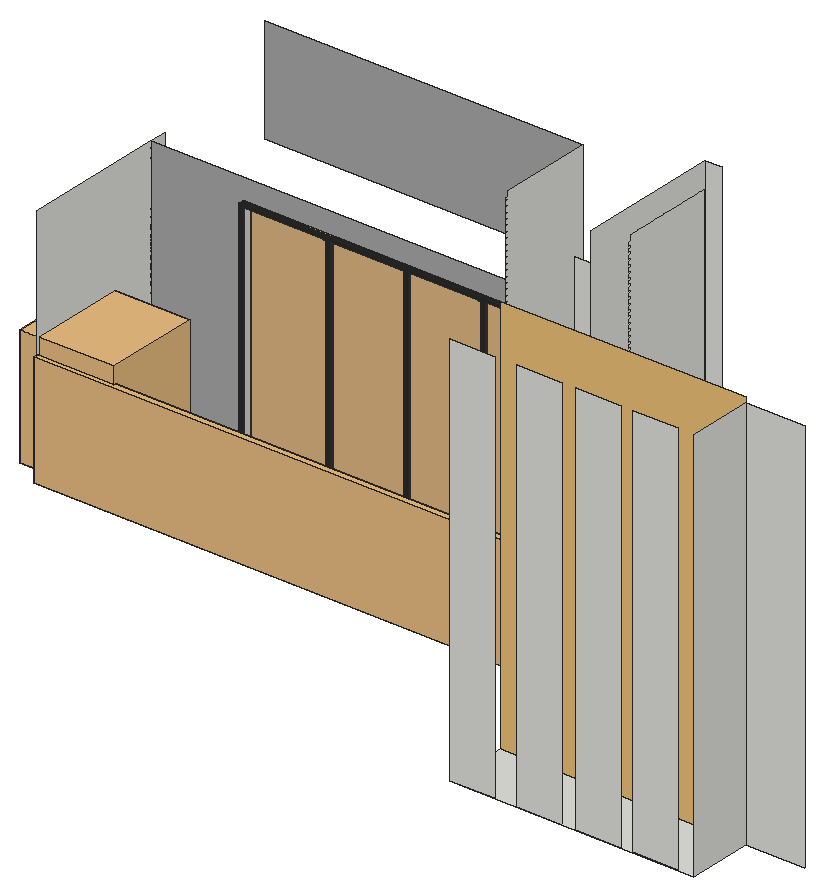
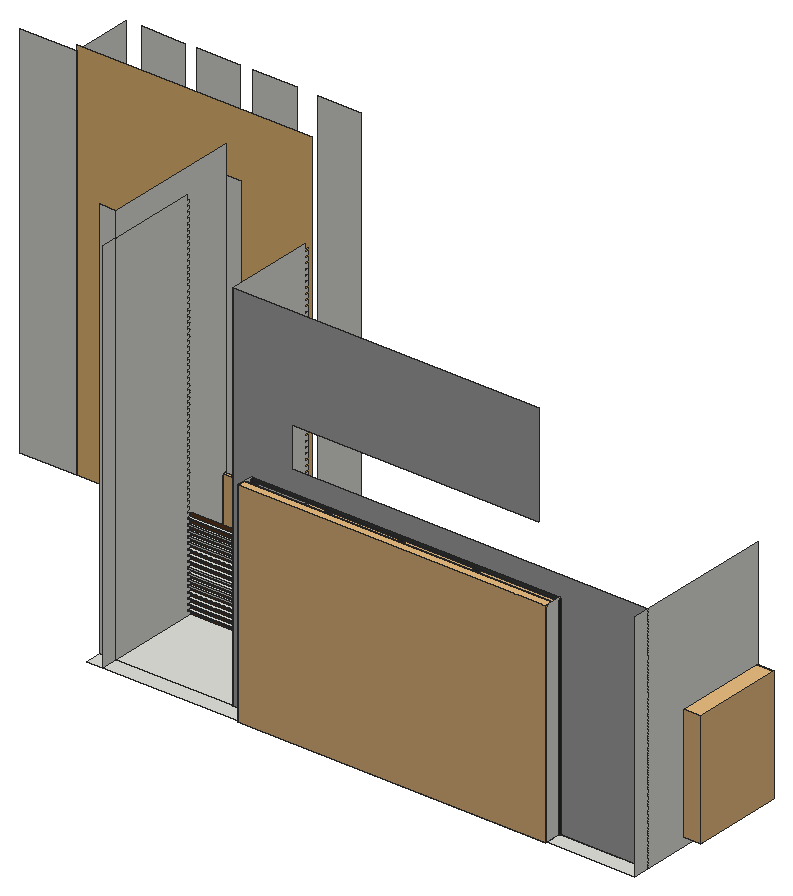
# SketchUp Ruby script. Lengths in inches.
U = 1.inch
M = Sketchup.active_model
def pt(a) = Geom::Point3d.new(a.map { |v| v * U })
def face(e, loops, mat)
  f = e.add_face(loops[0].map { |a| pt(a) })
  loops[1..].each { |l| e.add_face(l.map { |a| pt(a) }).erase! }
  f.material = f.back_material = mat if mat
  f
end
# faces: each face lists its corners as indices into pts; further lists are holes
def faces(e, pts, list, mat = nil) = list.each { |f| face(e, (f[0].is_a?(Array) ? f : [f]).map { |l| l.map { |i| pts[i] } }, mat) }
# xy, xz, yz: faces in a plane at the given z, y or x. An outline is a flat list of corners, or four numbers for a rectangle; further outlines are holes
def ring(l) = l.size == 4 ? [[l[0], l[1]], [l[2], l[1]], [l[2], l[3]], [l[0], l[3]]] : l.each_slice(2).to_a
def flat(e, list, mat, &to3) = list.each { |f| face(e, (f[0].is_a?(Array) ? f : [f]).map { |l| ring(l).map { |u, v| to3.(u, v) } }, mat) }
def xy(e, z, list, mat = nil) = flat(e, list, mat) { |x, y| [x, y, z] }
def xz(e, y, list, mat = nil) = flat(e, list, mat) { |x, z| [x, y, z] }
def yz(e, x, list, mat = nil) = flat(e, list, mat) { |y, z| [x, y, z] }
def lines(e, pts, list) = list.each { |a, b| e.add_line(pt(pts[a]), pt(pts[b])) }
# prism: a flat outline (further loops are holes) pulled along v
def prism(e, loops, v, mat = nil)
  f = face(e, loops, mat); d = Geom::Vector3d.new(v.map { |x| x * U })
  f.pushpull(f.normal.samedirection?(d) ? d.length : -d.length)
end
def box(e, o, s, mat = nil) = prism(e, [[o, [o[0] + s[0], o[1], o[2]], [o[0] + s[0], o[1] + s[1], o[2]], [o[0], o[1] + s[1], o[2]]]], [0, 0, s[2]], mat)
def at(x, y, z, deg = 0) = Geom::Transformation.translation(pt([x, y, z])) * Geom::Transformation.rotation(ORIGIN, Z_AXIS, deg.degrees)
def axes(o, x, y, z) = Geom::Transformation.new([*x, 0, *y, 0, *z, 0, *pt(o).to_a, 1])
def part(name) = M.definitions.add(name)
# library, detail: a bought-in or finely detailed component or shape, given as its bounding box
def library(name, o, s) = part(name).tap { |d| box(d.entities, o, s) }
def detail(e, o, s) = box(e.add_group.entities, o, s)
def put(e, d, t, mat = nil) = e.add_instance(d, t).tap { |i| i.material = mat if mat }
def group(e, t, mat = nil) = e.add_group.tap { |g| g.transformation = t; g.material = mat if mat }.entities
root = M.entities
M.materials.add("Glazing").color = [128, 128, 128]
M.materials["Glazing"].alpha = 0.05
M.materials.add("Powdercoating").color = [41, 44, 40]
M.materials.add("[Color M03]1").color = [170, 170, 170]
M.materials.add("[Wood OSB]1").color = [240, 195, 122]
M.materials.add("[Wood Veneer 01]").color = [96, 56, 29]
c1 = library("plant (1)",[-35.72,-28.42,0],[66.31,67.39,84.38])
c2 = part("Group\#15")
xy(c2.entities,0,[[0,-55.94,0.71,45.94]])
xy(c2.entities,0.2,[[0,-55.94,0.47,45.94],[0.47,45.94,0.71,46.42]])
xy(c2.entities,2.36,[[0.47,-55.94,0.71,46.42]])
xz(c2.entities,-55.94,[[0,0,0.71,0,0.71,2.36,0.47,2.36,0.47,0.2,0,0.2]])
xz(c2.entities,45.94,[[0,0,0.71,0.2]])
xz(c2.entities,46.42,[[0.47,0.2,0.71,2.36]])
yz(c2.entities,0,[[-55.94,0,45.94,0.2]])
yz(c2.entities,0.47,[[-55.94,0.2,46.42,2.36]])
yz(c2.entities,0.71,[[-55.94,0,45.94,0,45.94,0.2,46.42,0.2,46.42,2.36,-55.94,2.36]])
c3 = part("Group\#7")
xy(c3.entities,0,[[0,-59.09,0.71,45.94]])
xy(c3.entities,0.2,[[0,-59.09,0.47,45.94],[0.47,45.94,0.71,46.42]])
xy(c3.entities,2.36,[[0.47,-59.09,0.71,46.42]])
xz(c3.entities,-59.09,[[0,0,0.71,0,0.71,2.36,0.47,2.36,0.47,0.2,0,0.2]])
xz(c3.entities,45.94,[[0,0,0.71,0.2]])
xz(c3.entities,46.42,[[0.47,0.2,0.71,2.36]])
yz(c3.entities,0,[[-59.09,0,45.94,0.2]])
yz(c3.entities,0.47,[[-59.09,0.2,46.42,2.36]])
yz(c3.entities,0.71,[[-59.09,0,45.94,0,45.94,0.2,46.42,0.2,46.42,2.36,-59.09,2.36]])
c4 = part("Group\#16")
prism(c4.entities,[[[0.47,-56.18,0.2],[0,-56.18,0.2],[0,-56.18,0],[0.71,-56.18,0],[0.71,-56.18,2.36],[0.47,-56.18,2.36]]],[0,28.68,0])
c5 = part("Group\#10")
box(c5.entities,[-0.73,0,0],[27.99,0.55,102.05])
c6 = part("Group\#18")
xy(c6.entities,0,[[0.47,-56.18,0.47,-55.47,0,-55.47,0,-28.21,1.18,-28.21,1.18,-56.18]])
xy(c6.entities,0.2,[[0.71,-56.18,1.18,-28.21],[0,-55.47,0.47,-28.21],[0.47,-28.21,0.71,-27.74]])
xy(c6.entities,2.36,[[0.47,-56.18,0.71,-27.74]])
xz(c6.entities,-56.18,[[0.47,0,1.18,0,1.18,0.2,0.71,0.2,0.71,2.36,0.47,2.36]])
xz(c6.entities,-55.47,[[0,0,0.47,0.2]])
xz(c6.entities,-28.21,[[0,0,1.18,0.2]])
xz(c6.entities,-27.74,[[0.47,0.2,0.71,2.36]])
yz(c6.entities,0,[[-55.47,0,-28.21,0.2]])
yz(c6.entities,0.47,[[-56.18,0,-55.47,0.2],[-56.18,0.2,-27.74,2.36]])
yz(c6.entities,0.71,[[-56.18,0.2,-27.74,2.36]])
yz(c6.entities,1.18,[[-56.18,0,-28.21,0.2]])
c7 = part("Group\#34")
xy(c7.entities,0,[[-20.45,0,7.76,1.22]])
xy(c7.entities,0.06,[[-20.39,0.06,7.7,1.22]])
xy(c7.entities,0.47,[[-19.98,0,7.28,0.06]])
xy(c7.entities,101.89,[[-19.98,0,7.28,0.06]])
xy(c7.entities,102.3,[[-20.39,0.06,7.7,1.22]])
xy(c7.entities,102.36,[[-20.45,0,7.76,1.22]])
xz(c7.entities,0,[[[-20.45,0,7.76,102.36],[-19.98,0.47,7.28,101.89]]])
xz(c7.entities,0.06,[[[-20.39,0.06,7.7,102.3],[-19.98,0.47,7.28,101.89]]])
xz(c7.entities,1.22,[[[-20.45,0,7.76,102.36],[-20.39,0.06,7.7,102.3]]])
yz(c7.entities,-20.45,[[0,0,1.22,102.36]])
yz(c7.entities,-20.39,[[0.06,0.06,1.22,102.3]])
yz(c7.entities,-19.98,[[0,0.47,0.06,101.89]])
yz(c7.entities,7.28,[[0,0.47,0.06,101.89]])
yz(c7.entities,7.7,[[0.06,0.06,1.22,102.3]])
yz(c7.entities,7.76,[[0,0,1.22,102.36]])
c8 = part("Group\#6")
put(c8.entities,c2,axes([27.97,0,7.875],[1,0,0],[0,0,-1],[0,1,0]),"Powdercoating")
put(c8.entities,c3,axes([0.71,0,6.8],[-1,0,0],[0,0,-0.97687],[0,1,0]),"Powdercoating")
put(c8.entities,c4,axes([-27.5,0,-38.07],[0,0,-1],[-1,0,0],[0,1,0]),"Powdercoating")
put(c8.entities,c5,at(1.12,0.35,-38.39),"Glazing")
put(c8.entities,c6,axes([-27.5,0,63.35],[0,0,1],[-1,0,0],[0,1,0]),"Powdercoating")
put(c8.entities,c7,at(20.6875,1.0625,-38.54),"Powdercoating")
c9 = part("Component\#2")
put(c9.entities,c8,at(-1.18,4.5,38.86))
g1 = group(c9.entities,at(84.74,4.5,38.86))
put(g1,c2,axes([-27.97,0,7.875],[-1,0,0],[0,0,-1],[0,1,0]),"Powdercoating")
put(g1,c3,axes([-0.71,0,6.8],[1,0,0],[0,0,-0.97687],[0,1,0]),"Powdercoating")
put(g1,c4,axes([27.5,0,-38.07],[0,0,-1],[1,0,0],[0,1,0]),"Powdercoating")
put(g1,c5,axes([-1.12,0.35,-38.39],[-1,0,0],[0,1,0],[0,0,1]),"Glazing")
put(g1,c6,axes([27.5,0,63.35],[0,0,1],[1,0,0],[0,1,0]),"Powdercoating")
put(g1,c7,axes([-20.6875,1.0625,-38.54],[-1,0,0],[0,1,0],[0,0,1]),"Powdercoating")
g2 = group(c9.entities,at(56.0625,4.5,38.86))
put(g2,c2,axes([-27.97,0,7.875],[-1,0,0],[0,0,-1],[0,1,0]),"Powdercoating")
put(g2,c4,axes([27.5,0,-38.07],[0,0,-1],[1,0,0],[0,1,0]),"Powdercoating")
put(g2,c5,axes([-1.12,0.35,-38.39],[-1,0,0],[0,1,0],[0,0,1]),"Glazing")
put(g2,c6,axes([27.5,0,63.35],[0,0,1],[1,0,0],[0,1,0]),"Powdercoating")
put(g2,c7,axes([-20.6875,1.0625,-38.54],[-1,0,0],[0,1,0],[0,0,1]),"Powdercoating")
g3 = group(g2,at(-0.71,0,6.8),"Powdercoating")
xy(g3,-45.34,[[0.47,0.2,0.71,2.36]])
xy(g3,-44.88,[[0,0,0.71,0.2]])
xy(g3,57.73,[[0,0,0.71,0,0.71,2.36,0.47,2.36,0.47,0.2,0,0.2]])
xz(g3,0,[[0,-44.88,0.71,57.73]])
xz(g3,0.2,[[0.47,-45.34,0.71,-44.88],[0,-44.88,0.47,57.73]])
xz(g3,2.36,[[0.47,-45.34,0.71,57.73]])
yz(g3,0,[[0,-44.88,0.2,57.73]])
yz(g3,0.47,[[0.2,-45.34,2.36,57.73]])
yz(g3,0.71,[[0.2,-45.34,2.36,-45.34,2.36,57.73,0,57.73,0,-44.88,0.2,-44.88]])
put(c9.entities,c8,axes([-33.94,4.5,38.86],[1.14218,0,0],[0,1,0],[0,0,1]))
c10 = part("sliding door")
put(c10.entities,c9,at(0,-4.5,-0.08))
c11 = library("panneau+shadow+blanc+bourdon+naturel",[-47.99,-1.29,1.53],[97.82,5.86,114.18])
c12 = library("Glass Railing",[0,0,0],[139.5,4.76,42])
xy(root,191.19,[[609.34,322.97,782.78,368.59]])
xy(root,199,[[228.06,433.78,620.86,433.78,620.86,465.95,534.24,465.95,534.24,534.98,228.06,534.98],[534.24,465.95,620.86,534.98],[228.06,534.98,292.8,546.92],[292.8,534.98,520.24,546.92],[520.24,534.98,620.86,546.92],
  [620.86,534.98,632.79,546.92]])
xy(root,202.03,[[534.24,465.95,620.86,468.64]])
xy(root,202.9375,[[534.24,465.95,620.86,468.64]])
xy(root,205.97,[[534.24,465.95,620.86,468.64]])
xy(root,206.9375,[[534.24,465.95,620.86,468.64]])
xy(root,209.97,[[534.24,465.95,620.86,468.64]])
xy(root,211,[[534.24,465.95,620.86,468.64]])
xy(root,214.03,[[534.24,465.95,620.86,468.64]])
xy(root,215.0625,[[534.24,465.95,620.86,468.64]])
xy(root,218.09,[[534.24,465.95,620.86,468.64]])
xy(root,219.125,[[534.24,465.95,620.86,468.64]])
xy(root,222.16,[[534.24,465.95,620.86,468.64]])
xy(root,223.1875,[[534.24,465.95,620.86,468.64]])
xy(root,226.22,[[534.24,465.95,620.86,468.64]])
xy(root,227.25,[[534.24,465.95,620.86,468.64]])
xy(root,230.28,[[534.24,465.95,620.86,468.64]])
xy(root,231.3125,[[534.24,465.95,620.86,468.64]])
xy(root,234.34,[[534.24,465.95,620.86,468.64]])
xy(root,235.375,[[534.24,465.95,620.86,468.64]])
xy(root,238.41,[[534.24,465.95,620.86,468.64]])
xy(root,239.4375,[[534.24,465.95,620.86,468.64]])
xy(root,242.47,[[534.24,465.95,620.86,468.64]])
xy(root,243.5,[[534.24,465.95,620.86,468.64]])
xy(root,246.53,[[534.24,465.95,620.86,468.64]])
xy(root,247.5625,[[534.24,465.95,620.86,468.64]])
xy(root,250.59,[[534.24,465.95,620.86,468.64]])
xy(root,251.625,[[534.24,465.95,620.86,468.64]])
xy(root,254.66,[[534.24,465.95,620.86,468.64]])
xy(root,255.6875,[[534.24,466.33,620.86,468.64]])
xy(root,258.72,[[534.24,466.33,620.86,468.64]])
xy(root,259.75,[[534.24,466.33,620.86,468.64]])
xy(root,262.78,[[534.24,466.33,620.86,468.64]])
xy(root,263.8125,[[534.24,466.33,620.86,468.64]])
xz(root,322.97,[[609.34,191.19,641.55,471.94],[657.03,191.19,689.24,471.94],[698.65,191.19,730.86,471.94],[739.28,191.19,771.49,471.94]])
xz(root,368.59,[[782.78,191.19,824.53,471.94]])
xz(root,368.59,[[609.34,191.19,782.78,475.57]],"[Wood OSB]1")
xz(root,433.78,[[609.34,199,620.86,475.57]])
xz(root,465.95,[[534.24,199,620.86,202.03],[534.24,202.9375,620.86,205.97],[534.24,206.9375,620.86,209.97],[534.24,211,620.86,214.03],[534.24,215.0625,620.86,218.09],
  [534.24,219.125,620.86,222.16],[534.24,223.1875,620.86,226.22],[534.24,227.25,620.86,230.28],[534.24,231.3125,620.86,234.34],[534.24,235.375,620.86,238.41],
  [534.24,239.4375,620.86,242.47],[534.24,243.5,620.86,246.53],[534.24,247.5625,620.86,250.59],[534.24,251.625,620.86,254.66]],"[Wood Veneer 01]")
xz(root,466.33,[[534.24,255.6875,620.86,258.72],[534.24,259.75,620.86,262.78],[534.24,263.8125,620.86,266.84]],"[Wood Veneer 01]")
xz(root,468.64,[[534.24,202.03,620.86,202.9375],[534.24,205.97,620.86,206.9375],[534.24,209.97,620.86,211],[534.24,214.03,620.86,215.0625],[534.24,218.09,620.86,219.125],
  [534.24,222.16,620.86,223.1875],[534.24,226.22,620.86,227.25],[534.24,230.28,620.86,231.3125],[534.24,234.34,620.86,235.375],[534.24,238.41,620.86,239.4375],
  [534.24,242.47,620.86,243.5],[534.24,246.53,620.86,247.5625],[534.24,250.59,620.86,251.625],[534.24,254.66,620.86,255.6875],[534.24,258.72,620.86,259.75],
  [534.24,262.78,620.86,263.8125]])
xz(root,534.98,[[620.86,199,632.79,496.07]])
xz(root,534.98,[[228.06,199,292.8,199,292.8,355.625,520.24,355.625,520.24,199,534.24,199,534.24,475.57,308.65,475.57,308.65,400,490.99,400,490.99,370.64,228.06,370.64]],"[Color M03]1")
yz(root,228.06,[[433.78,199,534.98,370.64],[534.98,199,546.92,370.64]])
yz(root,292.8,[[534.98,199,546.92,355.625]])
yz(root,520.24,[[534.98,199,546.92,355.625]])
yz(root,534.24,[[465.95,199,465.95,202.03,468.64,202.03,468.64,202.9375,465.95,202.9375,465.95,205.97,468.64,205.97,468.64,206.9375,465.95,206.9375,465.95,209.97,468.64,209.97,468.64,211,465.95,211,465.95,214.03,468.64,214.03,468.64,215.0625,465.95,215.0625,465.95,218.09,468.64,218.09,468.64,219.125,465.95,219.125,465.95,222.16,468.64,222.16,468.64,223.1875,465.95,223.1875,465.95,226.22,468.64,226.22,468.64,227.25,465.95,227.25,465.95,230.28,468.64,230.28,468.64,231.3125,465.95,231.3125,465.95,234.34,468.64,234.34,468.64,235.375,465.95,235.375,465.95,238.41,468.64,238.41,468.64,239.4375,465.95,239.4375,465.95,242.47,468.64,242.47,468.64,243.5,465.95,243.5,465.95,246.53,468.64,246.53,468.64,247.5625,465.95,247.5625,465.95,250.59,468.64,250.59,468.64,251.625,465.95,251.625,465.95,254.66,468.64,254.66,468.64,255.6875,466.33,255.6875,466.33,258.72,468.64,258.72,468.64,259.75,466.33,259.75,466.33,262.78,468.64,262.78,468.64,263.8125,466.33,263.8125,466.33,266.84,468.64,266.84,468.64,267.875,466.33,267.875,466.33,270.91,468.64,270.91,468.64,271.9375,466.33,271.9375,466.33,274.97,468.64,274.97,468.64,276,466.33,276,466.33,279.03,468.64,279.03,468.64,280.0625,466.33,280.0625,466.33,283.09,468.64,283.09,468.64,284.125,466.33,284.125,466.33,287.16,468.64,287.16,468.64,288.1875,466.33,288.1875,466.33,291.22,468.64,291.22,468.64,292.25,466.33,292.25,466.33,295.28,468.64,295.28,468.64,296.3125,466.33,296.3125,466.33,299.34,468.64,299.34,468.64,300.375,466.33,300.375,466.33,303.41,468.64,303.41,468.64,304.4375,466.33,304.4375,466.33,307.47,468.64,307.47,468.64,308.5,466.33,308.5,466.33,311.53,468.64,311.53,468.64,312.5625,466.33,312.5625,466.33,315.59,468.64,315.59,468.64,316.625,466.33,316.625,466.33,319.66,468.64,319.66,468.64,320.6875,466.33,320.6875,466.33,323.72,468.64,323.72,468.64,324.75,466.33,324.75,466.33,327.78,468.64,327.78,468.64,328.8125,466.33,328.8125,466.33,331.84,468.64,331.84,468.64,332.875,466.33,332.875,466.33,335.91,468.64,335.91,468.64,336.9375,466.33,336.9375,466.33,339.97,468.64,339.97,468.64,341,466.33,341,466.33,344.03,468.64,344.03,468.64,345.0625,466.33,345.0625,466.33,348.09,468.64,348.09,468.64,349.125,466.33,349.125,466.33,352.16,468.64,352.16,468.64,353.1875,466.33,353.1875,466.33,356.22,468.64,356.22,468.64,357.25,466.33,357.25,466.33,360.28,468.64,360.28,468.64,361.3125,466.33,361.3125,466.33,364.34,468.64,364.34,468.64,365.375,466.33,365.375,466.33,368.41,468.64,368.41,468.64,369.4375,466.33,369.4375,466.33,372.47,468.64,372.47,468.64,373.5,466.33,373.5,466.33,376.53,468.64,376.53,468.64,377.5625,466.33,377.5625,466.33,380.59,468.64,380.59,468.64,381.625,466.33,381.625,466.33,384.66,468.64,384.66,468.64,385.6875,466.33,385.6875,466.33,388.72,468.64,388.72,468.64,389.75,466.33,389.75,466.33,392.78,468.64,392.78,468.64,393.8125,466.33,393.8125,466.33,396.84,468.64,396.84,468.64,397.875,466.33,397.875,466.33,400.91,468.64,400.91,468.64,401.9375,466.33,401.9375,466.33,404.97,468.64,404.97,468.64,406,466.33,406,466.33,409.03,468.64,409.03,468.64,410.0625,466.33,410.0625,466.33,413.09,468.64,413.09,468.64,414.125,466.33,414.125,466.33,417.16,468.64,417.16,468.64,418.1875,466.33,418.1875,466.33,421.22,468.64,421.22,468.64,422.25,466.33,422.25,466.33,425.28,468.64,425.28,468.64,426.3125,466.33,426.3125,466.33,429.34,468.64,429.34,468.64,430.375,466.33,430.375,466.33,433.41,468.64,433.41,468.64,434.4375,466.33,434.4375,466.33,437.47,468.64,437.47,468.64,438.5,466.33,438.5,466.33,441.53,468.64,441.53,468.64,442.5625,466.33,442.5625,466.33,445.59,468.64,445.59,468.64,446.625,466.33,446.625,466.33,449.66,468.64,449.66,468.64,450.6875,466.33,450.6875,466.33,453.72,468.64,453.72,468.64,454.75,466.33,454.75,466.33,457.78,468.64,457.78,468.64,458.8125,466.33,458.8125,466.33,461.84,468.64,461.84,468.64,462.875,466.33,462.875,466.33,465.91,468.64,465.91,468.64,466.9375,466.33,466.9375,466.33,469.97,468.64,469.97,468.64,471,466.33,471,466.33,471.94,468.64,471.94,468.64,475.57,534.98,475.57,534.98,199]])
yz(root,620.86,[[433.78,199,433.78,496.07,534.98,496.07,534.98,478.09,468.64,478.09,468.64,474.03,466.33,474.03,466.33,471,468.64,471,468.64,469.97,466.33,469.97,466.33,466.9375,468.64,466.9375,468.64,465.91,466.33,465.91,466.33,462.875,468.64,462.875,468.64,461.84,466.33,461.84,466.33,458.8125,468.64,458.8125,468.64,457.78,466.33,457.78,466.33,454.75,468.64,454.75,468.64,453.72,466.33,453.72,466.33,450.6875,468.64,450.6875,468.64,449.66,466.33,449.66,466.33,446.625,468.64,446.625,468.64,445.59,466.33,445.59,466.33,442.5625,468.64,442.5625,468.64,441.53,466.33,441.53,466.33,438.5,468.64,438.5,468.64,437.47,466.33,437.47,466.33,434.4375,468.64,434.4375,468.64,433.41,466.33,433.41,466.33,430.375,468.64,430.375,468.64,429.34,466.33,429.34,466.33,426.3125,468.64,426.3125,468.64,425.28,466.33,425.28,466.33,422.25,468.64,422.25,468.64,421.22,466.33,421.22,466.33,418.1875,468.64,418.1875,468.64,417.16,466.33,417.16,466.33,414.125,468.64,414.125,468.64,413.09,466.33,413.09,466.33,410.0625,468.64,410.0625,468.64,409.03,466.33,409.03,466.33,406,468.64,406,468.64,404.97,466.33,404.97,466.33,401.9375,468.64,401.9375,468.64,400.91,466.33,400.91,466.33,397.875,468.64,397.875,468.64,396.84,466.33,396.84,466.33,393.8125,468.64,393.8125,468.64,392.78,466.33,392.78,466.33,389.75,468.64,389.75,468.64,388.72,466.33,388.72,466.33,385.6875,468.64,385.6875,468.64,384.66,466.33,384.66,466.33,381.625,468.64,381.625,468.64,380.59,466.33,380.59,466.33,377.5625,468.64,377.5625,468.64,376.53,466.33,376.53,466.33,373.5,468.64,373.5,468.64,372.47,466.33,372.47,466.33,369.4375,468.64,369.4375,468.64,368.41,466.33,368.41,466.33,365.375,468.64,365.375,468.64,364.34,466.33,364.34,466.33,361.3125,468.64,361.3125,468.64,360.28,466.33,360.28,466.33,357.25,468.64,357.25,468.64,356.22,466.33,356.22,466.33,353.1875,468.64,353.1875,468.64,352.16,466.33,352.16,466.33,349.125,468.64,349.125,468.64,348.09,466.33,348.09,466.33,345.0625,468.64,345.0625,468.64,344.03,466.33,344.03,466.33,341,468.64,341,468.64,339.97,466.33,339.97,466.33,336.9375,468.64,336.9375,468.64,335.91,466.33,335.91,466.33,332.875,468.64,332.875,468.64,331.84,466.33,331.84,466.33,328.8125,468.64,328.8125,468.64,327.78,466.33,327.78,466.33,324.75,468.64,324.75,468.64,323.72,466.33,323.72,466.33,320.6875,468.64,320.6875,468.64,319.66,466.33,319.66,466.33,316.625,468.64,316.625,468.64,315.59,466.33,315.59,466.33,312.5625,468.64,312.5625,468.64,311.53,466.33,311.53,466.33,308.5,468.64,308.5,468.64,307.47,466.33,307.47,466.33,304.4375,468.64,304.4375,468.64,303.41,466.33,303.41,466.33,300.375,468.64,300.375,468.64,299.34,466.33,299.34,466.33,296.3125,468.64,296.3125,468.64,295.28,466.33,295.28,466.33,292.25,468.64,292.25,468.64,291.22,466.33,291.22,466.33,288.1875,468.64,288.1875,468.64,287.16,466.33,287.16,466.33,284.125,468.64,284.125,468.64,283.09,466.33,283.09,466.33,280.0625,468.64,280.0625,468.64,279.03,466.33,279.03,466.33,276,468.64,276,468.64,274.97,466.33,274.97,466.33,271.9375,468.64,271.9375,468.64,270.91,466.33,270.91,466.33,267.875,468.64,267.875,468.64,266.84,466.33,266.84,466.33,263.8125,468.64,263.8125,468.64,262.78,466.33,262.78,466.33,259.75,468.64,259.75,468.64,258.72,466.33,258.72,466.33,255.6875,468.64,255.6875,468.64,254.66,465.95,254.66,465.95,251.625,468.64,251.625,468.64,250.59,465.95,250.59,465.95,247.5625,468.64,247.5625,468.64,246.53,465.95,246.53,465.95,243.5,468.64,243.5,468.64,242.47,465.95,242.47,465.95,239.4375,468.64,239.4375,468.64,238.41,465.95,238.41,465.95,235.375,468.64,235.375,468.64,234.34,465.95,234.34,465.95,231.3125,468.64,231.3125,468.64,230.28,465.95,230.28,465.95,227.25,468.64,227.25,468.64,226.22,465.95,226.22,465.95,223.1875,468.64,223.1875,468.64,222.16,465.95,222.16,465.95,219.125,468.64,219.125,468.64,218.09,465.95,218.09,465.95,215.0625,468.64,215.0625,468.64,214.03,465.95,214.03,465.95,211,468.64,211,468.64,209.97,465.95,209.97,465.95,206.9375,468.64,206.9375,468.64,205.97,465.95,205.97,465.95,202.9375,468.64,202.9375,468.64,202.03,465.95,202.03,465.95,199],[465.95,199,465.95,202.03,468.64,202.03,468.64,202.9375,465.95,202.9375,465.95,205.97,468.64,205.97,468.64,206.9375,465.95,206.9375,465.95,209.97,468.64,209.97,468.64,211,465.95,211,465.95,214.03,468.64,214.03,468.64,215.0625,465.95,215.0625,465.95,218.09,468.64,218.09,468.64,219.125,465.95,219.125,465.95,222.16,468.64,222.16,468.64,223.1875,465.95,223.1875,465.95,226.22,468.64,226.22,468.64,227.25,465.95,227.25,465.95,230.28,468.64,230.28,468.64,231.3125,465.95,231.3125,465.95,234.34,468.64,234.34,468.64,235.375,465.95,235.375,465.95,238.41,468.64,238.41,468.64,239.4375,465.95,239.4375,465.95,242.47,468.64,242.47,468.64,243.5,465.95,243.5,465.95,246.53,468.64,246.53,468.64,247.5625,465.95,247.5625,465.95,250.59,468.64,250.59,468.64,251.625,465.95,251.625,465.95,254.66,468.64,254.66,468.64,255.6875,466.33,255.6875,466.33,258.72,468.64,258.72,468.64,259.75,466.33,259.75,466.33,262.78,468.64,262.78,468.64,263.8125,466.33,263.8125,466.33,266.84,468.64,266.84,468.64,267.875,466.33,267.875,466.33,270.91,468.64,270.91,468.64,271.9375,466.33,271.9375,466.33,274.97,468.64,274.97,468.64,276,466.33,276,466.33,279.03,468.64,279.03,468.64,280.0625,466.33,280.0625,466.33,283.09,468.64,283.09,468.64,284.125,466.33,284.125,466.33,287.16,468.64,287.16,468.64,288.1875,466.33,288.1875,466.33,291.22,468.64,291.22,468.64,292.25,466.33,292.25,466.33,295.28,468.64,295.28,468.64,296.3125,466.33,296.3125,466.33,299.34,468.64,299.34,468.64,300.375,466.33,300.375,466.33,303.41,468.64,303.41,468.64,304.4375,466.33,304.4375,466.33,307.47,468.64,307.47,468.64,308.5,466.33,308.5,466.33,311.53,468.64,311.53,468.64,312.5625,466.33,312.5625,466.33,315.59,468.64,315.59,468.64,316.625,466.33,316.625,466.33,319.66,468.64,319.66,468.64,320.6875,466.33,320.6875,466.33,323.72,468.64,323.72,468.64,324.75,466.33,324.75,466.33,327.78,468.64,327.78,468.64,328.8125,466.33,328.8125,466.33,331.84,468.64,331.84,468.64,332.875,466.33,332.875,466.33,335.91,468.64,335.91,468.64,336.9375,466.33,336.9375,466.33,339.97,468.64,339.97,468.64,341,466.33,341,466.33,344.03,468.64,344.03,468.64,345.0625,466.33,345.0625,466.33,348.09,468.64,348.09,468.64,349.125,466.33,349.125,466.33,352.16,468.64,352.16,468.64,353.1875,466.33,353.1875,466.33,356.22,468.64,356.22,468.64,357.25,466.33,357.25,466.33,360.28,468.64,360.28,468.64,361.3125,466.33,361.3125,466.33,364.34,468.64,364.34,468.64,365.375,466.33,365.375,466.33,368.41,468.64,368.41,468.64,369.4375,466.33,369.4375,466.33,372.47,468.64,372.47,468.64,373.5,466.33,373.5,466.33,376.53,468.64,376.53,468.64,377.5625,466.33,377.5625,466.33,380.59,468.64,380.59,468.64,381.625,466.33,381.625,466.33,384.66,468.64,384.66,468.64,385.6875,466.33,385.6875,466.33,388.72,468.64,388.72,468.64,389.75,466.33,389.75,466.33,392.78,468.64,392.78,468.64,393.8125,466.33,393.8125,466.33,396.84,468.64,396.84,468.64,397.875,466.33,397.875,466.33,400.91,468.64,400.91,468.64,401.9375,466.33,401.9375,466.33,404.97,468.64,404.97,468.64,406,466.33,406,466.33,409.03,468.64,409.03,468.64,410.0625,466.33,410.0625,466.33,413.09,468.64,413.09,468.64,414.125,466.33,414.125,466.33,417.16,468.64,417.16,468.64,418.1875,466.33,418.1875,466.33,421.22,468.64,421.22,468.64,422.25,466.33,422.25,466.33,425.28,468.64,425.28,468.64,426.3125,466.33,426.3125,466.33,429.34,468.64,429.34,468.64,430.375,466.33,430.375,466.33,433.41,468.64,433.41,468.64,434.4375,466.33,434.4375,466.33,437.47,468.64,437.47,468.64,438.5,466.33,438.5,466.33,441.53,468.64,441.53,468.64,442.5625,466.33,442.5625,466.33,445.59,468.64,445.59,468.64,446.625,466.33,446.625,466.33,449.66,468.64,449.66,468.64,450.6875,466.33,450.6875,466.33,453.72,468.64,453.72,468.64,454.75,466.33,454.75,466.33,457.78,468.64,457.78,468.64,458.8125,466.33,458.8125,466.33,461.84,468.64,461.84,468.64,462.875,466.33,462.875,466.33,465.91,468.64,465.91,468.64,466.9375,466.33,466.9375,466.33,469.97,468.64,469.97,468.64,471,466.33,471,466.33,474.03,468.64,474.03,468.64,478.09,534.98,478.09,534.98,199],[534.98,199,546.92,478.09]])
yz(root,782.78,[[322.97,191.19,368.59,471.94]])
put(root,c1,at(250.94,463.43,205.73))
put(root,c10,axes([357.55,532.65,198.7],[1.9177,0,0],[0,1.51,0],[0,0,1.51]))
put(root,c11,axes([404.39,543.34,196.89],[2.32508,0,0],[0,1,0],[0,0,1.37182]))
put(root,c12,axes([228.06,431.36,198.94],[2.81576,0,0],[0,1,0],[0,0,1.9]))
